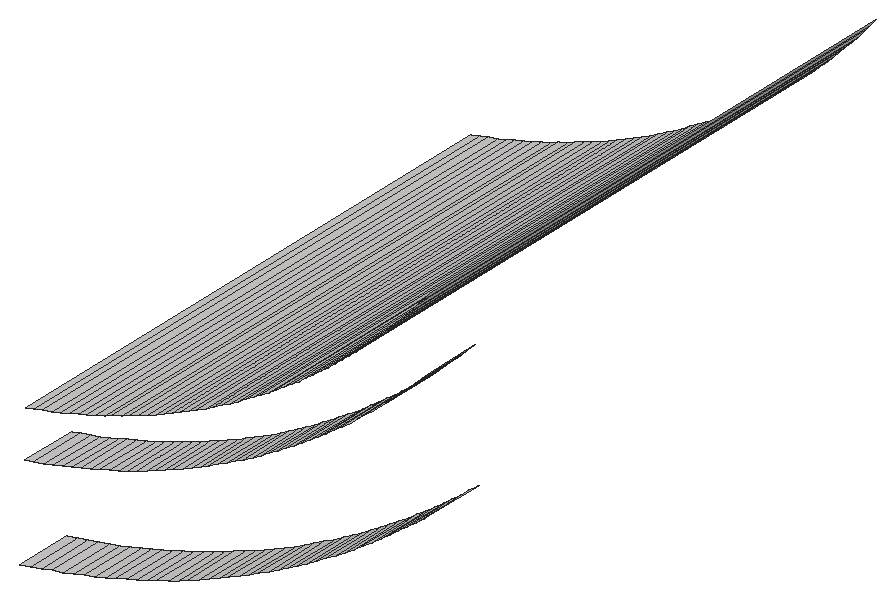
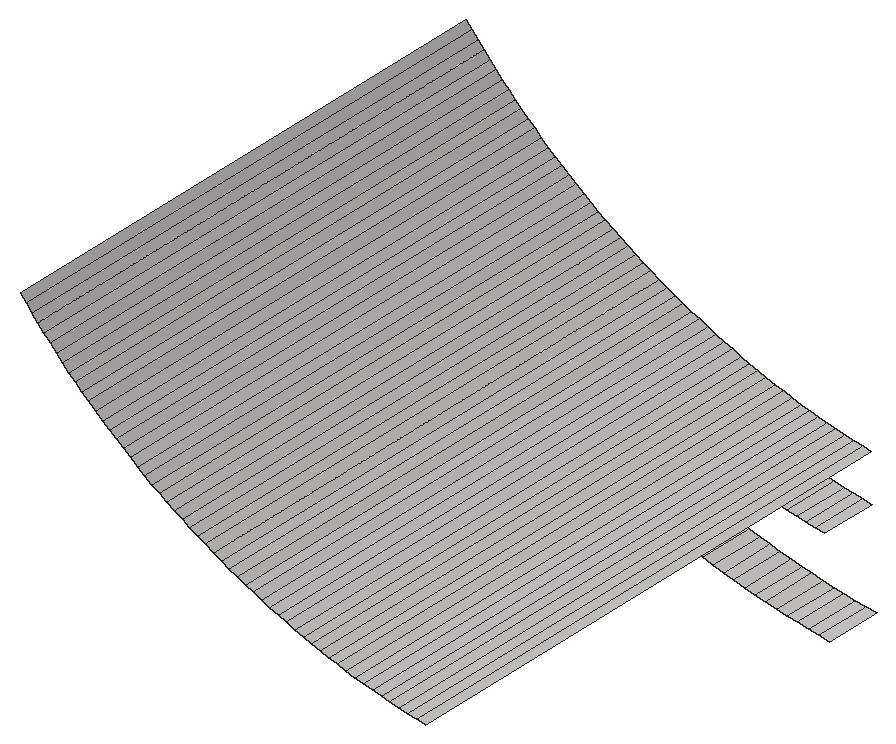
# SketchUp Ruby script. Lengths in inches.
U = 1.inch
M = Sketchup.active_model
def pt(a) = Geom::Point3d.new(a.map { |v| v * U })
def face(e, loops, mat)
  f = e.add_face(loops[0].map { |a| pt(a) })
  loops[1..].each { |l| e.add_face(l.map { |a| pt(a) }).erase! }
  f.material = f.back_material = mat if mat
  f
end
# faces: each face lists its corners as indices into pts; further lists are holes
def faces(e, pts, list, mat = nil) = list.each { |f| face(e, (f[0].is_a?(Array) ? f : [f]).map { |l| l.map { |i| pts[i] } }, mat) }
# xy, xz, yz: faces in a plane at the given z, y or x. An outline is a flat list of corners, or four numbers for a rectangle; further outlines are holes
def ring(l) = l.size == 4 ? [[l[0], l[1]], [l[2], l[1]], [l[2], l[3]], [l[0], l[3]]] : l.each_slice(2).to_a
def flat(e, list, mat, &to3) = list.each { |f| face(e, (f[0].is_a?(Array) ? f : [f]).map { |l| ring(l).map { |u, v| to3.(u, v) } }, mat) }
def xy(e, z, list, mat = nil) = flat(e, list, mat) { |x, y| [x, y, z] }
def xz(e, y, list, mat = nil) = flat(e, list, mat) { |x, z| [x, y, z] }
def yz(e, x, list, mat = nil) = flat(e, list, mat) { |y, z| [x, y, z] }
def lines(e, pts, list) = list.each { |a, b| e.add_line(pt(pts[a]), pt(pts[b])) }
# prism: a flat outline (further loops are holes) pulled along v
def prism(e, loops, v, mat = nil)
  f = face(e, loops, mat); d = Geom::Vector3d.new(v.map { |x| x * U })
  f.pushpull(f.normal.samedirection?(d) ? d.length : -d.length)
end
def box(e, o, s, mat = nil) = prism(e, [[o, [o[0] + s[0], o[1], o[2]], [o[0] + s[0], o[1] + s[1], o[2]], [o[0], o[1] + s[1], o[2]]]], [0, 0, s[2]], mat)
def at(x, y, z, deg = 0) = Geom::Transformation.translation(pt([x, y, z])) * Geom::Transformation.rotation(ORIGIN, Z_AXIS, deg.degrees)
def axes(o, x, y, z) = Geom::Transformation.new([*x, 0, *y, 0, *z, 0, *pt(o).to_a, 1])
def part(name) = M.definitions.add(name)
# library, detail: a bought-in or finely detailed component or shape, given as its bounding box
def library(name, o, s) = part(name).tap { |d| box(d.entities, o, s) }
def detail(e, o, s) = box(e.add_group.entities, o, s)
def put(e, d, t, mat = nil) = e.add_instance(d, t).tap { |i| i.material = mat if mat }
def group(e, t, mat = nil) = e.add_group.tap { |g| g.transformation = t; g.material = mat if mat }.entities
root = M.entities
M.materials.add("[Quartz Light Brown]").color = [215, 212, 212]
p = [[452.82,144.25,150.22],[452.82,143,150.22],[453.05,143,150.26],[453.05,144.25,150.26],[453.28,143,150.3],[453.28,144.25,150.3],
  [453.51,143,150.35],[453.51,144.25,150.35],[453.74,143,150.39],[453.74,144.25,150.39],[453.97,143,150.44],[453.97,144.25,150.44],
  [454.2,143,150.5],[454.2,144.25,150.5],[454.43,143,150.55],[454.43,144.25,150.55],[454.66,143,150.61],[454.66,144.25,150.61],
  [454.89,143,150.68],[454.89,144.25,150.68],[455.11,143,150.74],[455.11,144.25,150.74],[455.34,143,150.81],[455.34,144.25,150.81],
  [455.5625,143,150.88],[455.5625,144.25,150.88],[455.79,143,150.96],[455.79,144.25,150.96],[456.01,143,151.03],[456.01,144.25,151.03],
  [456.23,143,151.11],[456.23,144.25,151.11],[456.45,143,151.2],[456.45,144.25,151.2],[456.67,143,151.28],[456.67,144.25,151.28],
  [456.89,143,151.37],[456.89,144.25,151.37],[457.11,143,151.46],[457.11,144.25,151.46],[457.32,143,151.56],[457.32,144.25,151.56],
  [457.54,143,151.65],[457.54,144.25,151.65],[457.75,143,151.75],[457.75,144.25,151.75],[457.96,143,151.86],[457.96,144.25,151.86],
  [458.17,143,151.96],[458.17,144.25,151.96],[458.38,143,152.07],[458.38,144.25,152.07],[458.59,143,152.18],[458.59,144.25,152.18],
  [458.8,143,152.3],[458.8,144.25,152.3],[453.12,143,152.31],[452.92,143,152.27],[452.92,144.25,152.27],[453.12,144.25,152.31],
  [453.33,143,152.35],[453.33,144.25,152.35],[453.53,143,152.39],[453.53,144.25,152.39],[459,143,152.41],[459,144.25,152.41],
  [453.74,143,152.44],[453.74,144.25,152.44],[453.9375,143,152.49],[453.9375,144.25,152.49],[459.2,143,152.53],[459.2,144.25,152.53],
  [454.14,143,152.55],[454.14,144.25,152.55],[454.34,143,152.6],[454.34,144.25,152.6],[459.4,143,152.65],[459.4,144.25,152.65],
  [454.54,143,152.66],[454.54,144.25,152.66],[454.74,143,152.72],[454.74,144.25,152.72],[454.94,143,152.78],[454.94,144.25,152.78],
  [459.61,143,152.78],[459.61,144.25,152.78],[455.14,143,152.85],[455.14,144.25,152.85],[455.34,143,152.92],[455.34,144.25,152.92],
  [459.8,143,152.9],[459.8,144.25,152.9],[455.54,143,152.99],[455.54,144.25,152.99],[460,143,153.03],[460,144.25,153.03],
  [455.73,143,153.0625],[455.73,144.25,153.0625],[460.2,143,153.17],[460.2,144.25,153.17],[455.93,143,153.14],[455.93,144.25,153.14],
  [456.12,143,153.22],[456.12,144.25,153.22],[456.32,143,153.3],[456.32,144.25,153.3],[460.39,143,153.3],[460.39,144.25,153.3],
  [452.93,143,153.29],[453.12,143,153.33],[453.12,155,153.33],[452.93,155,153.29],[453.31,143,153.37],[453.31,155,153.37],
  [456.51,143,153.38],[456.51,144.25,153.38],[460.58,143,153.4375],[460.58,144.25,153.4375],[453.5,143,153.41],[453.5,155,153.41],
  [453.69,143,153.46],[453.69,155,153.46],[456.7,143,153.47],[456.7,144.25,153.47],[460.77,143,153.58],[460.77,144.25,153.58],
  [453.88,143,153.51],[453.88,155,153.51],[454.07,143,153.5625],[454.07,155,153.5625],[456.89,143,153.56],[456.89,144.25,153.56],
  [454.26,143,153.62],[454.26,155,153.62],[454.45,143,153.67],[454.45,155,153.67],[457.08,143,153.65],[457.08,144.25,153.65],
  [460.96,143,153.72],[460.96,144.25,153.72],[454.64,143,153.73],[454.64,155,153.73],[454.82,143,153.8],[454.82,155,153.8],
  [457.26,143,153.74],[457.26,144.25,153.74],[457.45,143,153.84],[457.45,144.25,153.84],[461.14,143,153.86],[461.14,144.25,153.86],
  [455.01,143,153.86],[455.01,155,153.86],[457.63,143,153.9375],[457.63,144.25,153.9375],[455.19,143,153.93],[455.19,155,153.93],
  [455.375,143,154],[455.375,155,154],[457.82,143,154.04],[457.82,144.25,154.04],[461.33,143,154.01],[461.33,144.25,154.01],
  [455.56,143,154.07],[455.56,155,154.07],[458,143,154.14],[458,144.25,154.14],[461.51,143,154.16],[461.51,144.25,154.16],
  [455.74,143,154.14],[455.74,155,154.14],[455.92,143,154.22],[455.92,155,154.22],[458.18,143,154.25],[458.18,144.25,154.25],
  [456.1,143,154.3],[456.1,155,154.3],[458.36,143,154.36],[458.36,144.25,154.36],[461.69,143,154.3125],[461.69,144.25,154.3125],
  [456.28,143,154.38],[456.28,155,154.38],[456.46,143,154.46],[456.46,155,154.46],[458.54,143,154.47],[458.54,144.25,154.47],
  [456.63,143,154.55],[456.63,155,154.55],[456.81,143,154.63],[456.81,155,154.63],[458.71,143,154.58],[458.71,144.25,154.58],
  [456.98,143,154.73],[456.98,155,154.73],[458.89,143,154.7],[458.89,144.25,154.7],[457.16,143,154.82],[457.16,155,154.82],
  [459.0625,143,154.8125],[459.0625,144.25,154.8125],[457.33,143,154.91],[457.33,155,154.91],[459.23,143,154.93],[459.23,144.25,154.93],
  [457.5,143,155.01],[457.5,155,155.01],[459.4,143,155.06],[459.4,144.25,155.06],[457.67,143,155.11],[457.67,155,155.11],
  [457.84,143,155.21],[457.84,155,155.21],[459.57,143,155.18],[459.57,144.25,155.18],[458,143,155.3125],[458,155,155.3125],
  [459.74,143,155.31],[459.74,144.25,155.31],[458.17,143,155.42],[458.17,155,155.42],[459.91,143,155.43],[459.91,144.25,155.43],
  [458.33,143,155.53],[458.33,155,155.53],[460.07,143,155.57],[460.07,144.25,155.57],[458.5,143,155.64],[458.5,155,155.64],
  [458.66,143,155.75],[458.66,155,155.75],[460.23,143,155.7],[460.23,144.25,155.7],[460.39,143,155.83],[460.39,144.25,155.83],
  [458.82,143,155.86],[458.82,155,155.86],[460.55,143,155.97],[460.55,144.25,155.97],[458.97,143,155.98],[458.97,155,155.98],
  [459.13,143,156.1],[459.13,155,156.1],[460.71,143,156.11],[460.71,144.25,156.11],[459.29,143,156.22],[459.29,155,156.22],
  [460.86,143,156.25],[460.86,144.25,156.25],[459.44,143,156.34],[459.44,155,156.34],[459.59,143,156.47],[459.59,155,156.47],
  [461.01,143,156.39],[461.01,144.25,156.39],[461.16,143,156.54],[461.16,144.25,156.54],[459.74,143,156.59],[459.74,155,156.59],
  [461.3125,143,156.6875],[461.3125,144.25,156.6875],[459.89,143,156.72],[459.89,155,156.72],[460.04,143,156.85],[460.04,155,156.85],
  [461.46,143,156.84],[461.46,144.25,156.84],[461.61,143,156.99],[461.61,144.25,156.99],[460.18,143,156.99],[460.18,155,156.99],
  [460.33,143,157.12],[460.33,155,157.12],[460.47,143,157.26],[460.47,155,157.26],[460.61,143,157.39],[460.61,155,157.39],
  [460.74,143,157.53],[460.74,155,157.53],[460.88,143,157.67],[460.88,155,157.67],[461.01,143,157.82],[461.01,155,157.82],
  [461.15,143,157.96],[461.15,155,157.96],[461.28,143,158.11],[461.28,155,158.11],[461.41,143,158.26],[461.41,155,158.26],
  [461.53,143,158.41],[461.53,155,158.41],[461.66,143,158.56],[461.66,155,158.56]]
faces(root,p,[[0,1,2,3],[3,2,4,5],[5,4,6,7],[7,6,8,9],[9,8,10,11],[11,10,12,13],[13,12,14,15],[15,14,16,17],
  [17,16,18,19],[19,18,20,21],[21,20,22,23],[23,22,24,25],[25,24,26,27],[27,26,28,29],[29,28,30,31],[31,30,32,33],
  [33,32,34,35],[35,34,36,37],[37,36,38,39],[39,38,40,41],[41,40,42,43],[43,42,44,45],[45,44,46,47],[47,46,48,49],
  [49,48,50,51],[51,50,52,53],[53,52,54,55],[56,57,58,59],[60,56,59,61],[62,60,61,63],[55,54,64,65],[66,62,63,67],
  [68,66,67,69],[65,64,70,71],[72,68,69,73],[74,72,73,75],[71,70,76,77],[78,74,75,79],[80,78,79,81],[82,80,81,83],
  [77,76,84,85],[86,82,83,87],[88,86,87,89],[85,84,90,91],[92,88,89,93],[91,90,94,95],[96,92,93,97],[95,94,98,99],
  [100,96,97,101],[102,100,101,103],[104,102,103,105],[99,98,106,107],[108,109,110,111],[109,112,113,110],[114,104,105,115],[107,106,116,117],
  [112,118,119,113],[118,120,121,119],[122,114,115,123],[117,116,124,125],[120,126,127,121],[126,128,129,127],[130,122,123,131],[128,132,133,129],
  [132,134,135,133],[136,130,131,137],[125,124,138,139],[134,140,141,135],[140,142,143,141],[144,136,137,145],[146,144,145,147],[139,138,148,149],
  [142,150,151,143],[152,146,147,153],[150,154,155,151],[154,156,157,155],[158,152,153,159],[149,148,160,161],[156,162,163,157],[164,158,159,165],
  [161,160,166,167],[162,168,169,163],[168,170,171,169],[172,164,165,173],[170,174,175,171],[176,172,173,177],[167,166,178,179],[174,180,181,175],
  [180,182,183,181],[184,176,177,185],[182,186,187,183],[186,188,189,187],[190,184,185,191],[188,192,193,189],[194,190,191,195],[192,196,197,193],
  [198,194,195,199],[196,200,201,197],[202,198,199,203],[200,204,205,201],[206,202,203,207],[204,208,209,205],[208,210,211,209],[212,206,207,213],
  [210,214,215,211],[216,212,213,217],[214,218,219,215],[220,216,217,221],[218,222,223,219],[224,220,221,225],[222,226,227,223],[226,228,229,227],
  [230,224,225,231],[232,230,231,233],[228,234,235,229],[236,232,233,237],[234,238,239,235],[238,240,241,239],[242,236,237,243],[240,244,245,241],
  [246,242,243,247],[244,248,249,245],[248,250,251,249],[252,246,247,253],[254,252,253,255],[250,256,257,251],[258,254,255,259],[256,260,261,257],
  [260,262,263,261],[264,258,259,265],[266,264,265,267],[262,268,269,263],[268,270,271,269],[270,272,273,271],[272,274,275,273],[274,276,277,275],
  [276,278,279,277],[278,280,281,279],[280,282,283,281],[282,284,285,283],[284,286,287,285],[286,288,289,287],[288,290,291,289]],"[Quartz Light Brown]")
